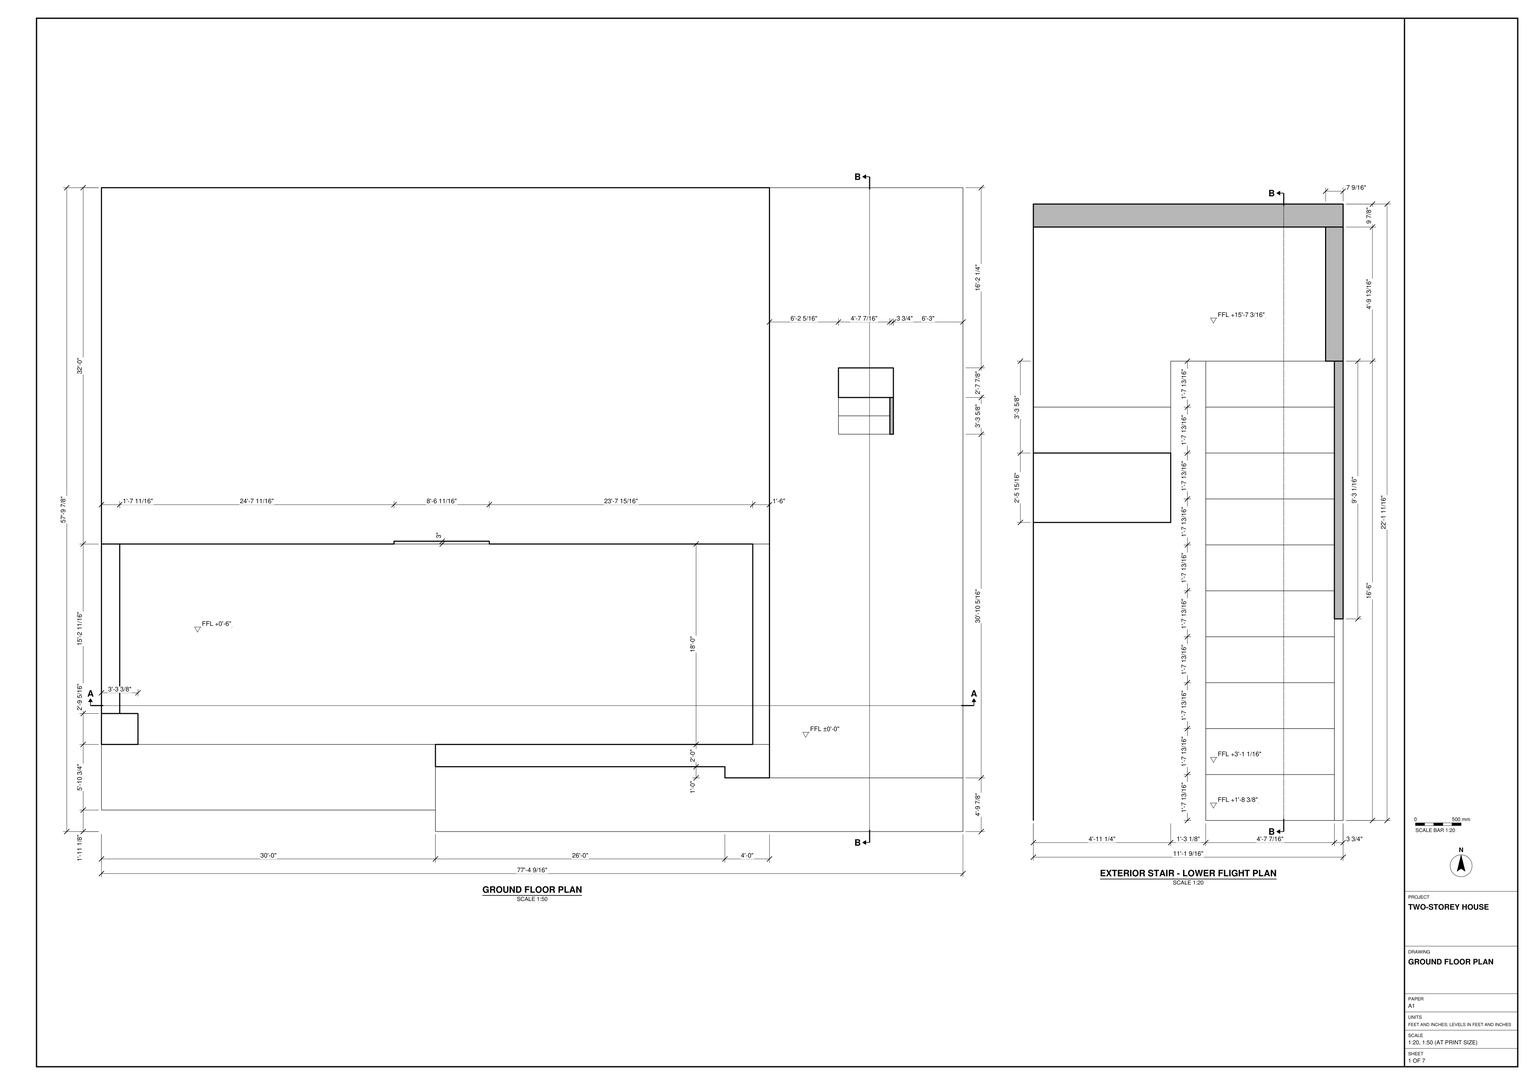
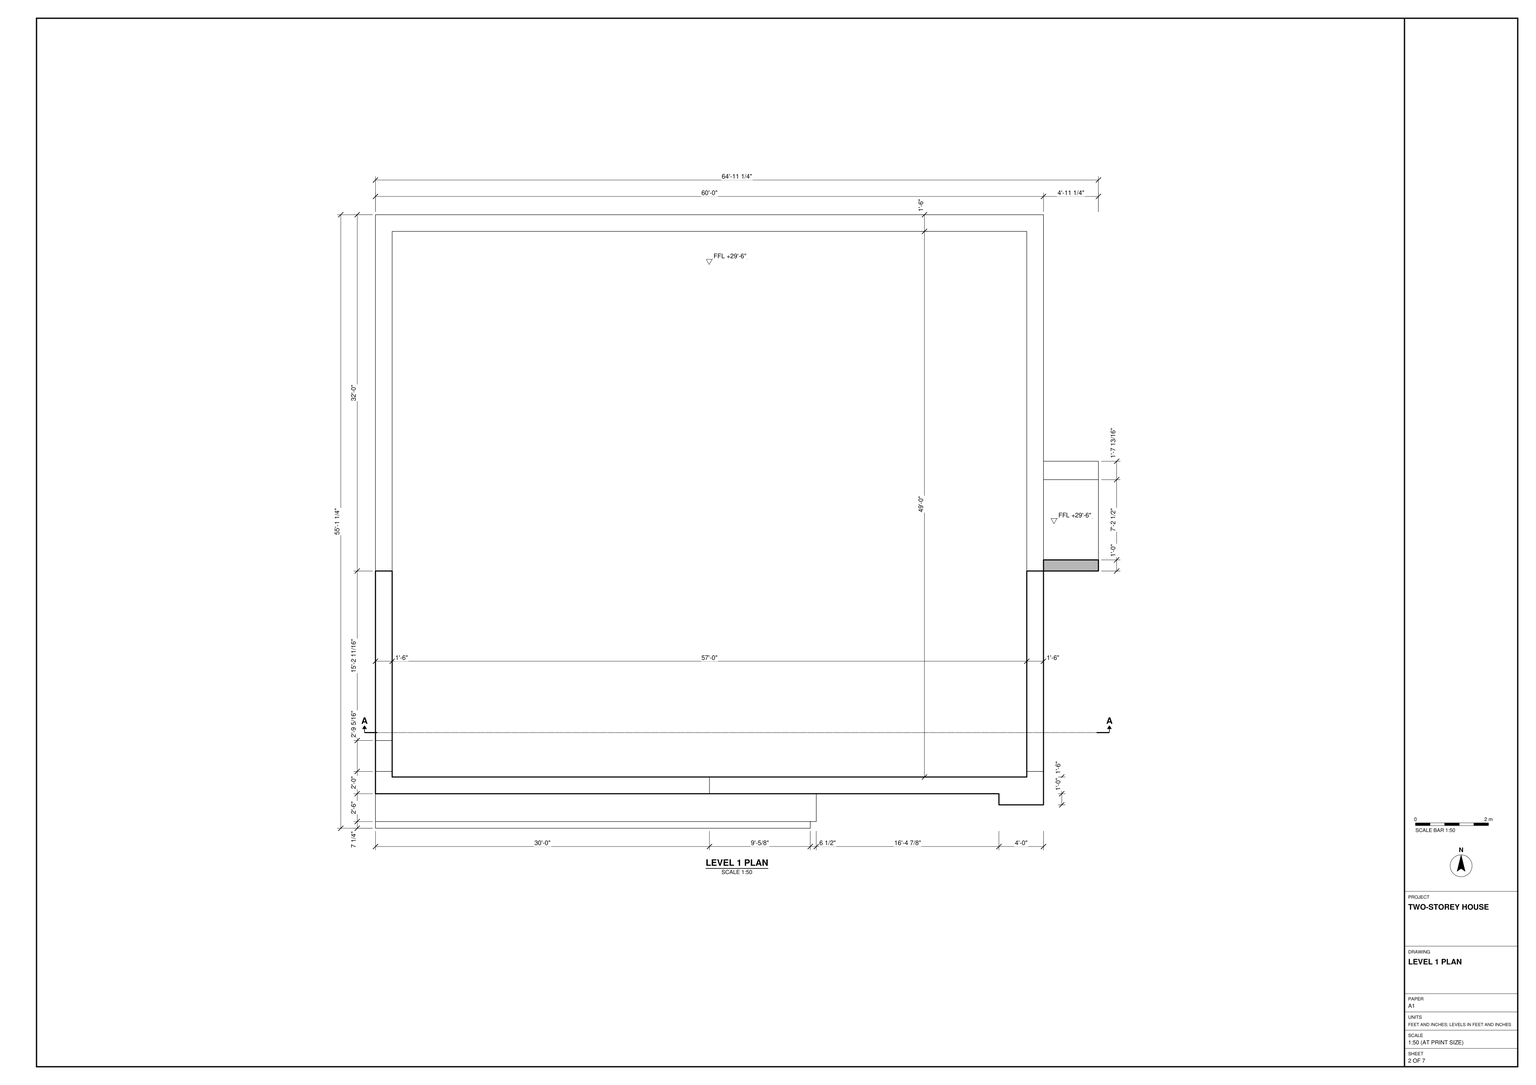
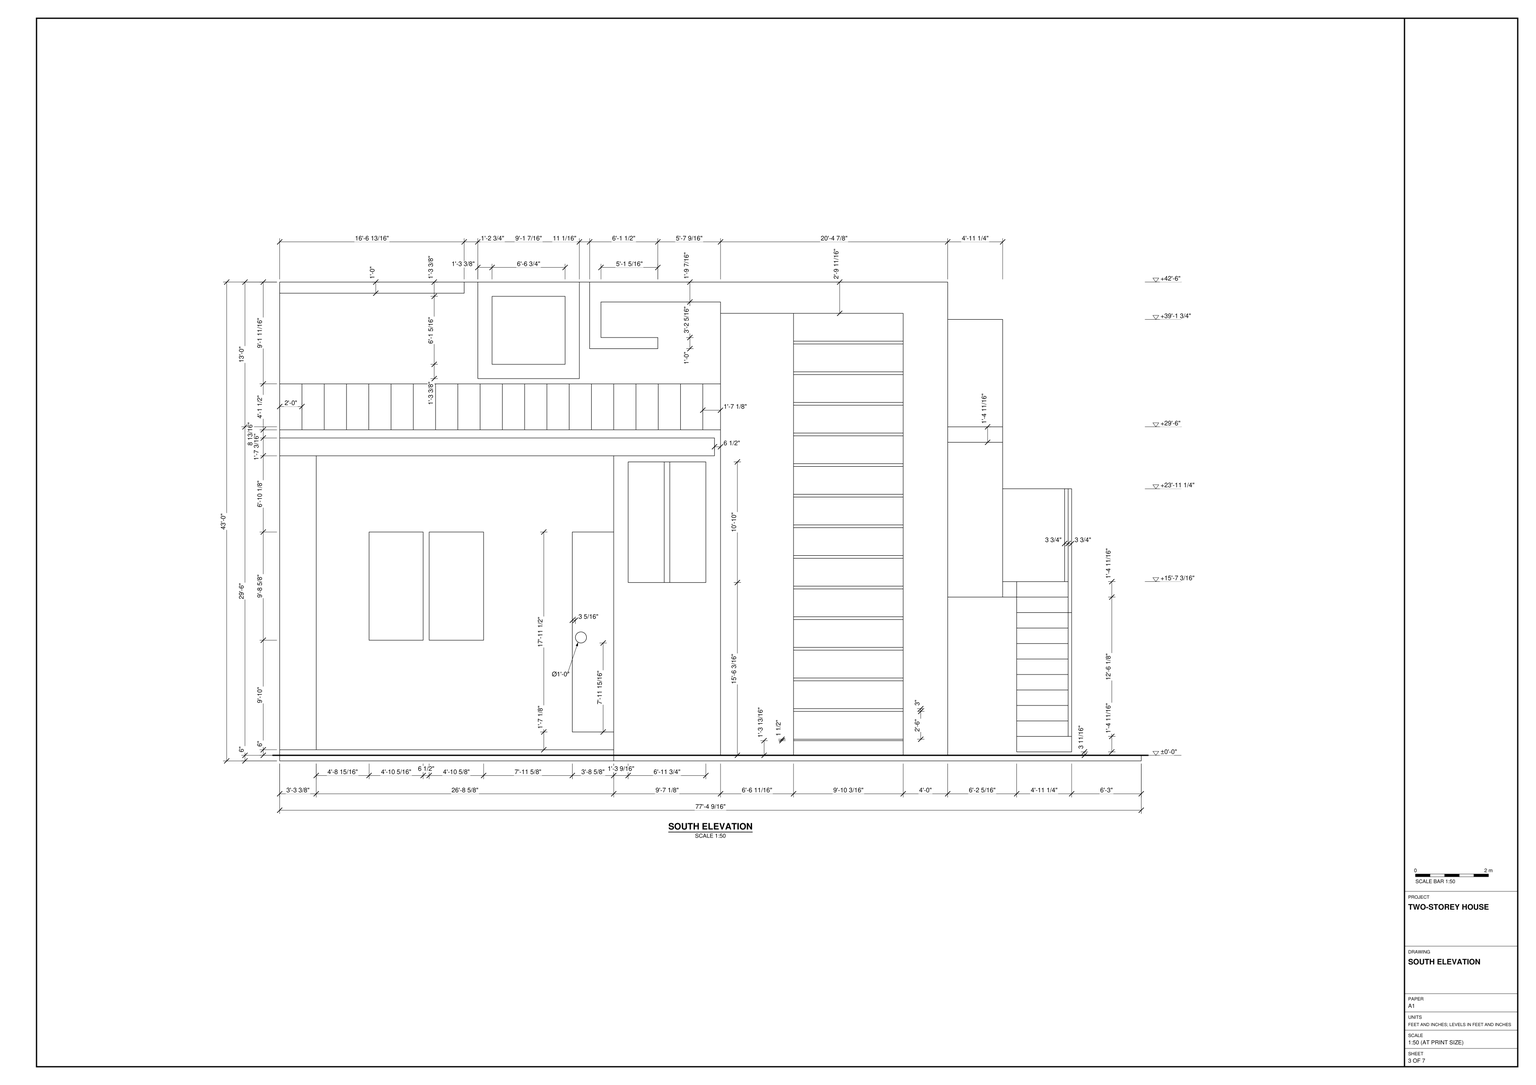
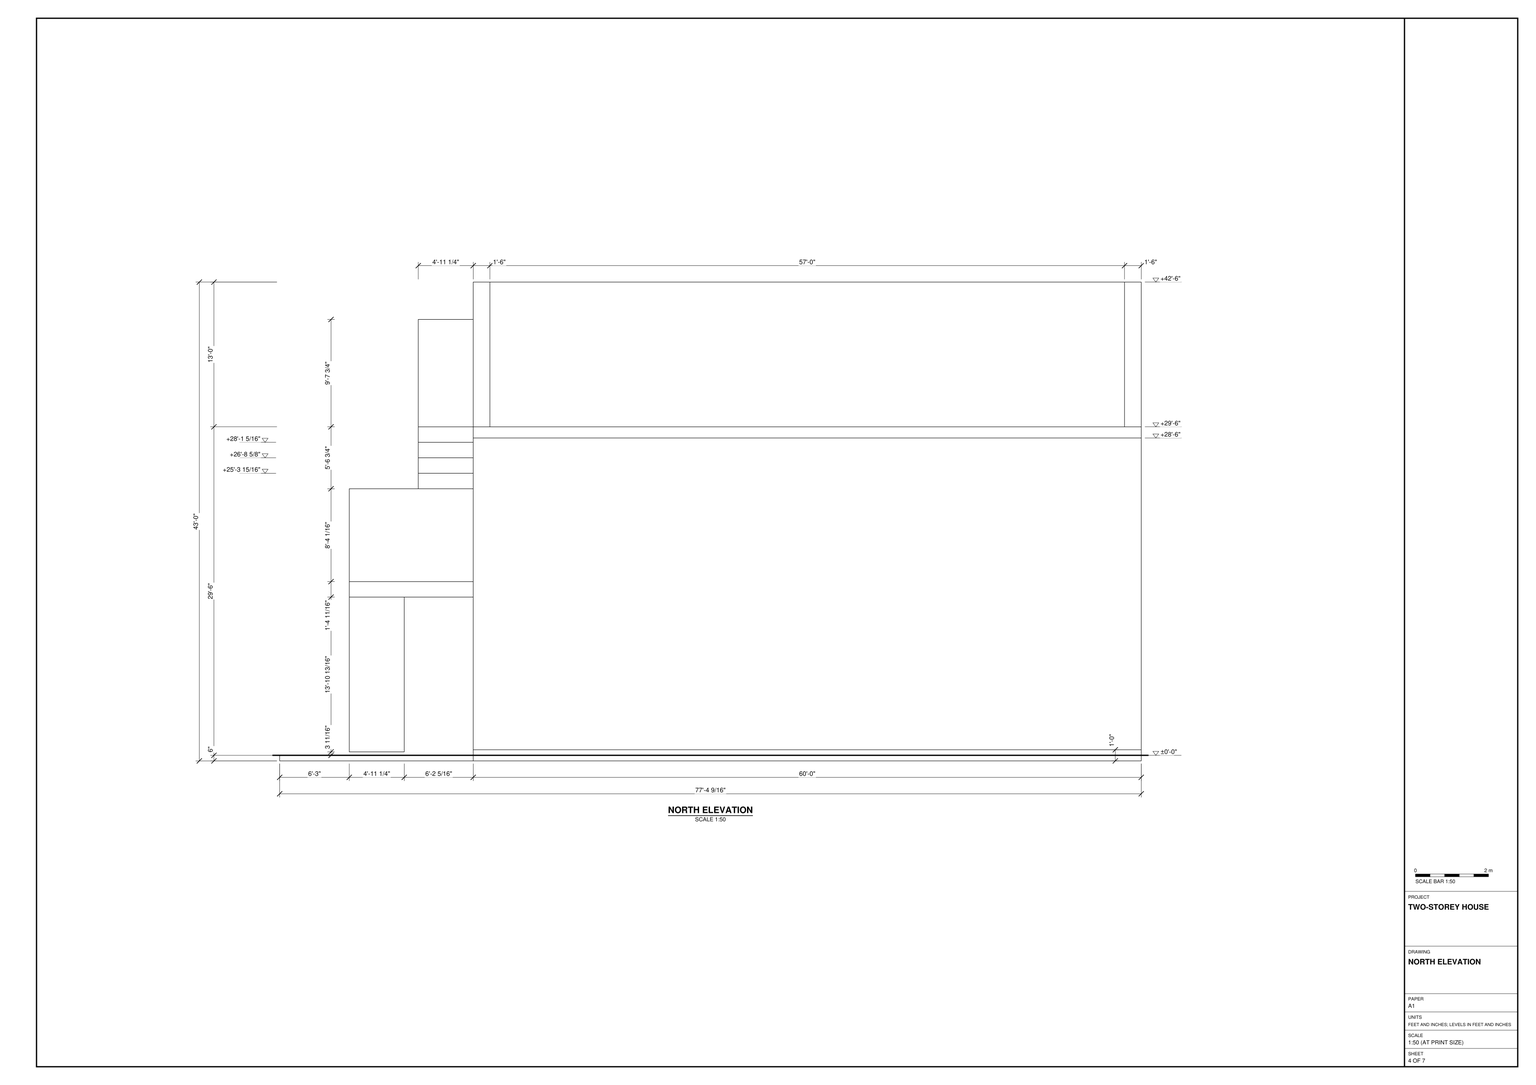
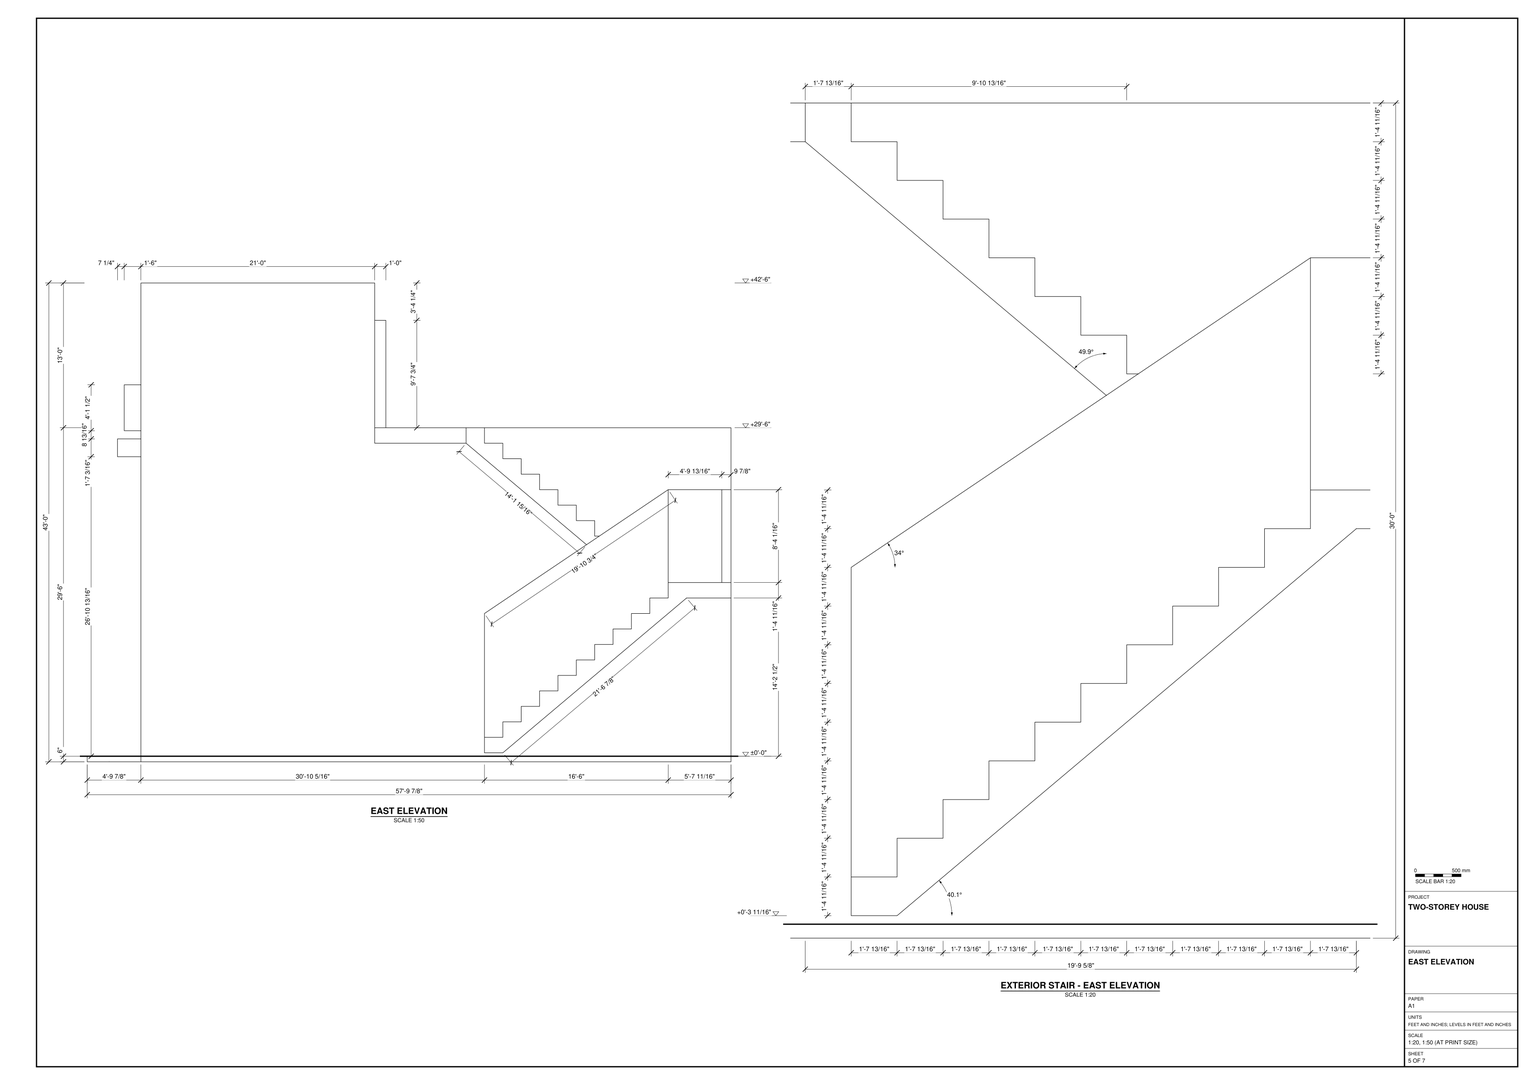
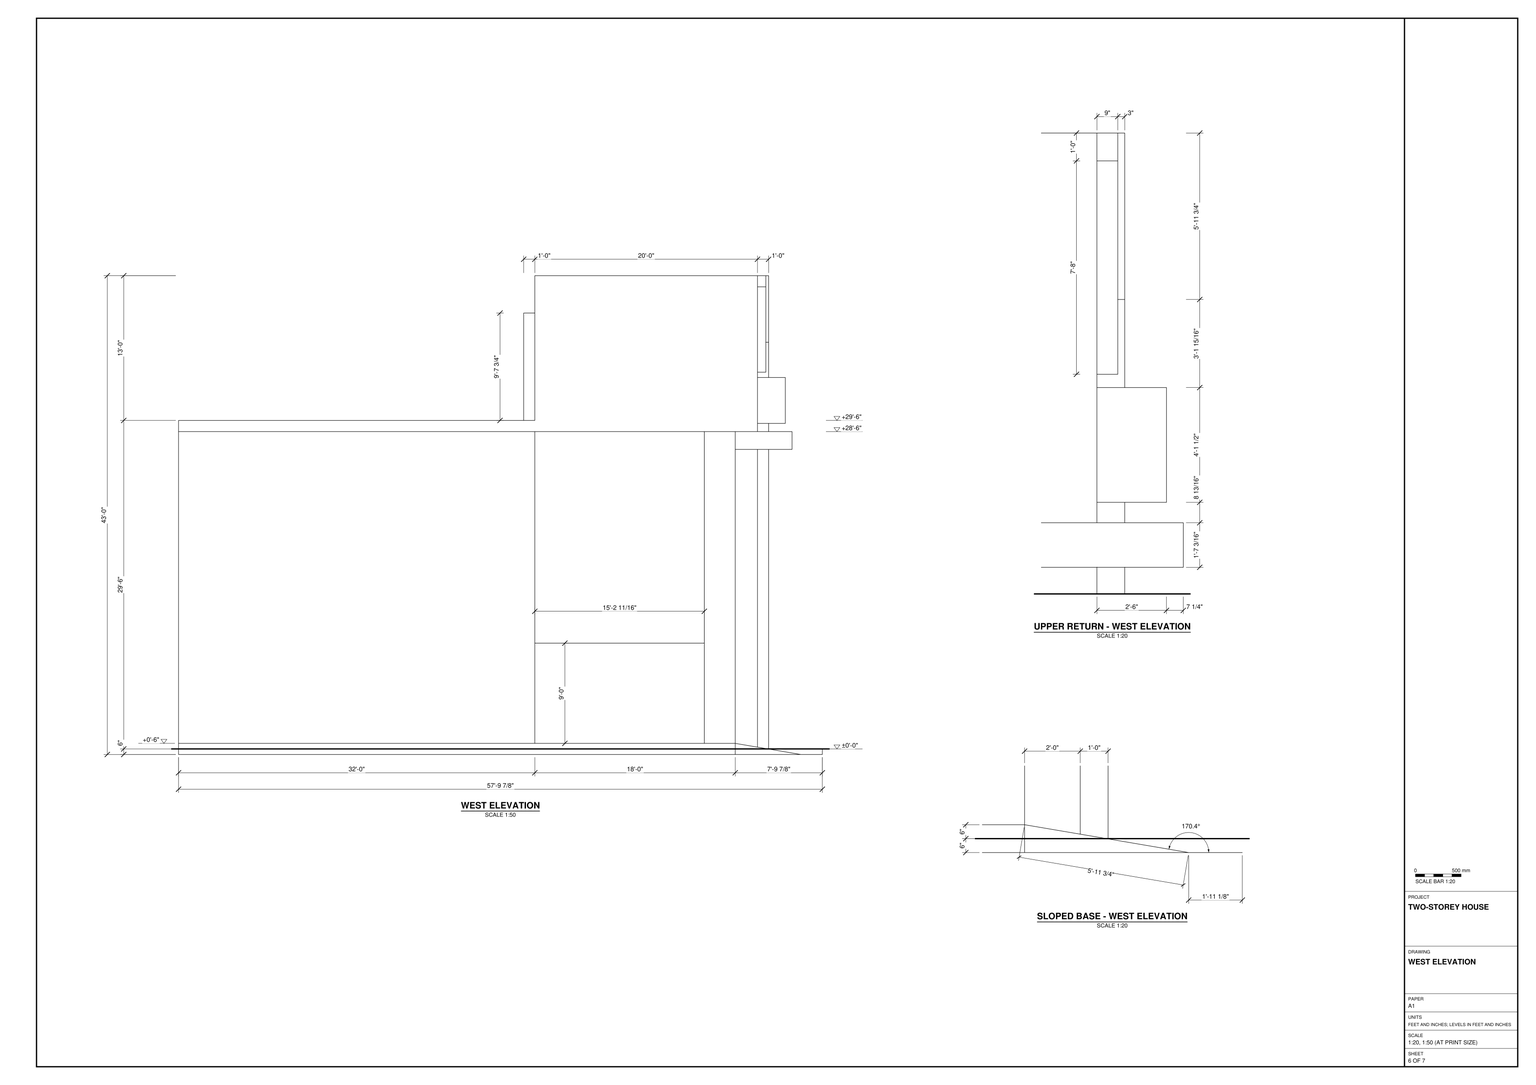
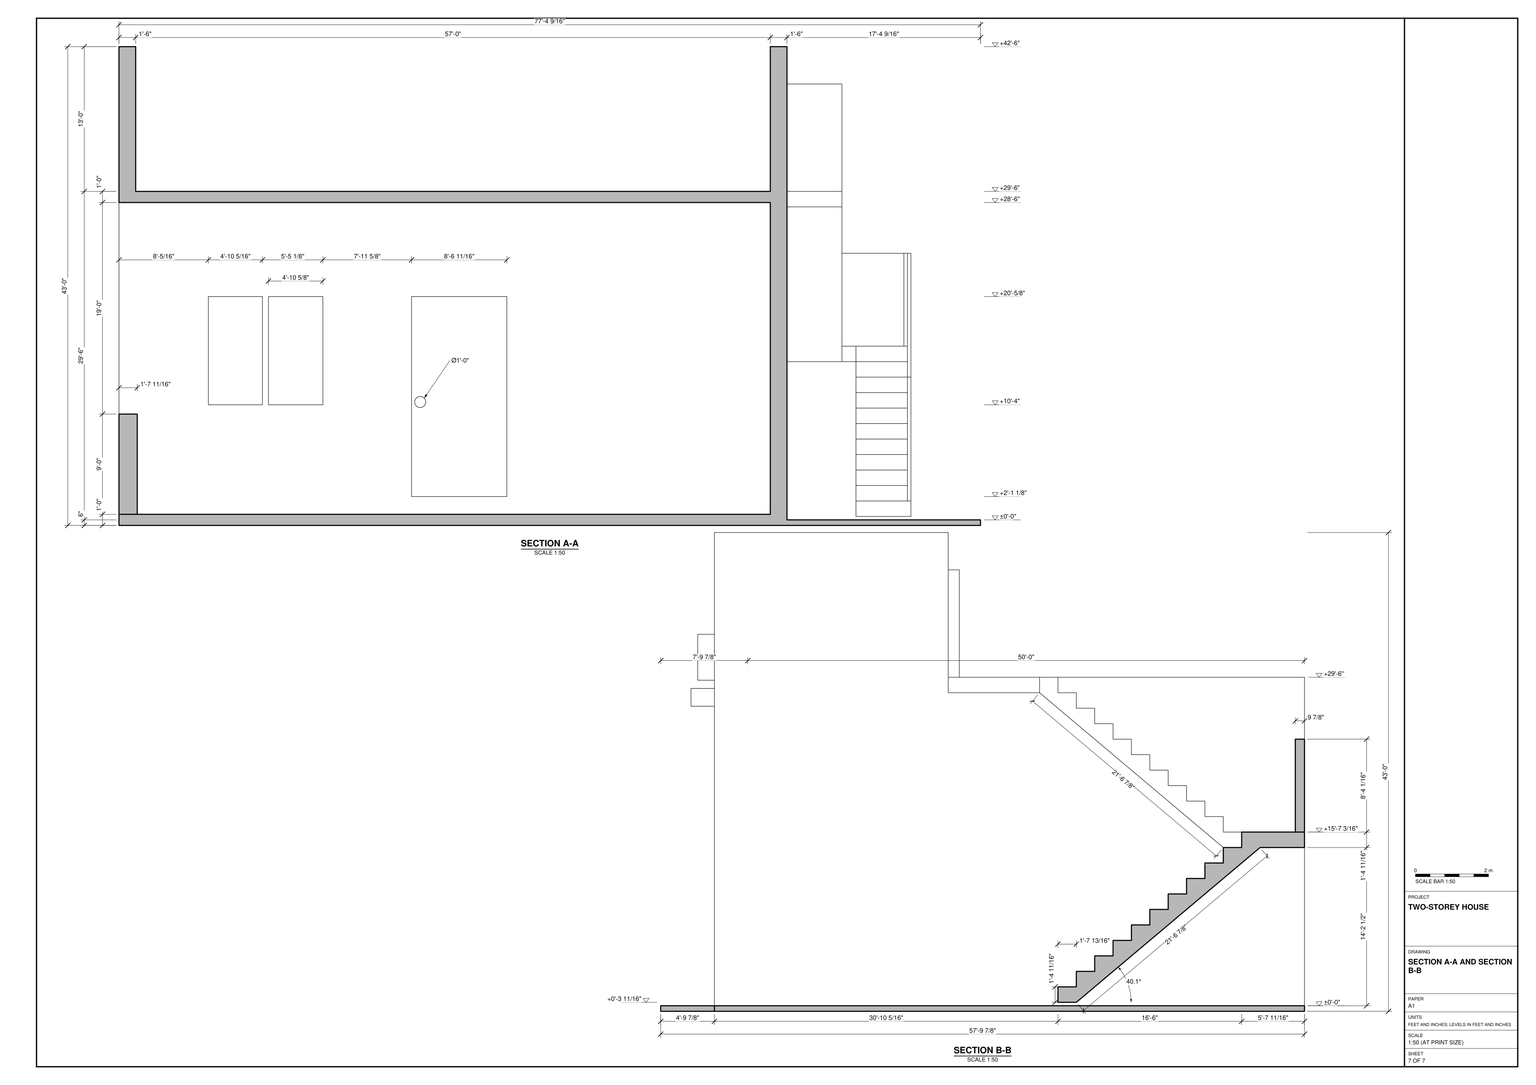
Build the house in SketchUp from task_files/diagram_01.pdf. Work in feet and inches. The overall model, including the base and exterior stair, measures 77'-4 9/16" along X, 57'-9 7/8" along Y and 43'-0" along Z. Set the ground-floor datum at ±0'-0" and the upper floor at +29'-6".

Use the plans to lay out the base, the recessed south frontage and the space beside the house for the stair. Model the walls at their drawn thicknesses and follow the slab edges, offsets and flat roof profile. On the south side, set the entrance wall back behind the outer support and horizontal beam. Place the door and window openings using the elevation, preserving the different sill heights. Model the divided band above the entrance, the square frame and adjoining angular detail near the roofline, and the tall horizontally banded bay toward the stair end of the facade.

Use the stair detail to set out the individual treads, side wall and intermediate landing. Align the return flight with the landing projecting from the upper floor. Keep walls, slabs, stairs and roof in separate groups or components, and group each furniture or joinery piece separately where shown. Use components for repeated parts. Decor and loose items, if shown, may use any suitable library component. Save one SketchUp model as output_files/two_storey_house_with_an_exterior_stair.skp.

# SketchUp Ruby script. Lengths in inches.
U = 1.inch
M = Sketchup.active_model
def pt(a) = Geom::Point3d.new(a.map { |v| v * U })
def face(e, loops, mat)
  f = e.add_face(loops[0].map { |a| pt(a) })
  loops[1..].each { |l| e.add_face(l.map { |a| pt(a) }).erase! }
  f.material = f.back_material = mat if mat
  f
end
# faces: each face lists its corners as indices into pts; further lists are holes
def faces(e, pts, list, mat = nil) = list.each { |f| face(e, (f[0].is_a?(Array) ? f : [f]).map { |l| l.map { |i| pts[i] } }, mat) }
# xy, xz, yz: faces in a plane at the given z, y or x. An outline is a flat list of corners, or four numbers for a rectangle; further outlines are holes
def ring(l) = l.size == 4 ? [[l[0], l[1]], [l[2], l[1]], [l[2], l[3]], [l[0], l[3]]] : l.each_slice(2).to_a
def flat(e, list, mat, &to3) = list.each { |f| face(e, (f[0].is_a?(Array) ? f : [f]).map { |l| ring(l).map { |u, v| to3.(u, v) } }, mat) }
def xy(e, z, list, mat = nil) = flat(e, list, mat) { |x, y| [x, y, z] }
def xz(e, y, list, mat = nil) = flat(e, list, mat) { |x, z| [x, y, z] }
def yz(e, x, list, mat = nil) = flat(e, list, mat) { |y, z| [x, y, z] }
def lines(e, pts, list) = list.each { |a, b| e.add_line(pt(pts[a]), pt(pts[b])) }
# prism: a flat outline (further loops are holes) pulled along v
def prism(e, loops, v, mat = nil)
  f = face(e, loops, mat); d = Geom::Vector3d.new(v.map { |x| x * U })
  f.pushpull(f.normal.samedirection?(d) ? d.length : -d.length)
end
def box(e, o, s, mat = nil) = prism(e, [[o, [o[0] + s[0], o[1], o[2]], [o[0] + s[0], o[1] + s[1], o[2]], [o[0], o[1] + s[1], o[2]]]], [0, 0, s[2]], mat)
def at(x, y, z, deg = 0) = Geom::Transformation.translation(pt([x, y, z])) * Geom::Transformation.rotation(ORIGIN, Z_AXIS, deg.degrees)
def axes(o, x, y, z) = Geom::Transformation.new([*x, 0, *y, 0, *z, 0, *pt(o).to_a, 1])
def part(name) = M.definitions.add(name)
# library, detail: a bought-in or finely detailed component or shape, given as its bounding box
def library(name, o, s) = part(name).tap { |d| box(d.entities, o, s) }
def detail(e, o, s) = box(e.add_group.entities, o, s)
def put(e, d, t, mat = nil) = e.add_instance(d, t).tap { |i| i.material = mat if mat }
def group(e, t, mat = nil) = e.add_group.tap { |g| g.transformation = t; g.material = mat if mat }.entities
root = M.entities
M.materials.add("[0006_Pink]").color = [255, 192, 203]
M.materials.add("[0007_MistyRose]").color = [255, 228, 225]
M.materials.add("[0009_Linen]").color = [250, 240, 230]
M.materials.add("[0018_Brown]").color = [79, 20, 20]
M.materials.add("[0099_LightSteelBlue]").color = [176, 196, 222]
M.materials.add("[0100_SteelBlue]").color = [60, 112, 155]
M.materials.add("[0110_LightSlateGray]").color = [119, 136, 153]
M.materials.add("[0118_Thistle]").color = [216, 191, 216]
M.materials.add("[0119_RosyBrown]").color = [188, 143, 143]
M.materials.add("[0125_Plum]").color = [221, 160, 221]
M.materials.add("[0137_Black]").color = [0, 0, 0]
M.materials.add("[Granite Dark Gray]").color = [69, 68, 68]
M.materials.add("[Grass Dark Green]").color = [106, 157, 55]
M.materials.add("[Stone Coursed Rough]").color = [165, 160, 130]
M.materials.add("[Stone Marble]").color = [143, 138, 136]
M.materials.add("[Translucent Glass Gray]").color = [128, 128, 128]
M.materials["[Translucent Glass Gray]"].alpha = 0.5
xy(root,0,[[360,0,928.5625,57.875],[0,23.125,360,93.875],[672,57.875,672,69.875,360,69.875,360,93.875,0,93.875,0,693.875,928.5625,693.875,928.5625,57.875],[360,57.875,672,69.875]])
xy(root,6,[[720,57.875,928.5625,693.875]])
xy(root,6,[[360,0,928.5625,0,928.5625,57.875,672,57.875,672,69.875,360,69.875]],"[Grass Dark Green]")
xy(root,9.69,[[794.34,428.16,853.56,447.96]])
xy(root,12,[[0,93.875,39.375,127.1875],[0,127.1875,19.6875,309.875]])
xy(root,12,[[39.375,93.875,702,93.875,702,309.875,19.6875,309.875,19.6875,127.1875,39.375,127.1875]],"[Stone Marble]")
xy(root,26.37,[[849.78,428.16,853.56,447.96]])
xy(root,26.37,[[794.34,428.16,849.78,447.96]],"[Granite Dark Gray]")
xy(root,31.15,[[315.37,309.875,418.06,312.875]])
xy(root,43.05,[[849.78,447.96,853.56,467.76]])
xy(root,43.05,[[794.34,447.96,849.78,467.76]],"[Granite Dark Gray]")
xy(root,59.73,[[849.78,467.76,853.56,487.56]])
xy(root,59.73,[[794.34,467.76,849.78,487.56]],"[Granite Dark Gray]")
xy(root,76.42,[[849.78,487.56,853.56,507.36]])
xy(root,76.42,[[794.34,487.56,849.78,507.36]],"[Granite Dark Gray]")
xy(root,93.1,[[849.78,507.36,853.56,527.16]])
xy(root,93.1,[[794.34,507.36,849.78,527.16]],"[Granite Dark Gray]")
xy(root,109.78,[[849.78,527.16,853.56,546.96]])
xy(root,109.78,[[794.34,527.16,849.78,546.96]],"[Granite Dark Gray]")
xy(root,120,[[0,127.1875,19.6875,309.875]])
xy(root,126.46,[[849.78,546.96,853.56,566.76]])
xy(root,126.46,[[794.34,546.96,849.78,566.76]],"[Granite Dark Gray]")
xy(root,130.02,[[96.32,309.875,154.63,311.875],[161.1,309.875,219.76,311.875]],"[0137_Black]")
xy(root,143.14,[[849.78,566.76,853.56,586.56]])
xy(root,143.14,[[794.34,566.76,849.78,586.56]],"[Granite Dark Gray]")
xy(root,159.82,[[849.78,586.56,853.56,606.36]])
xy(root,159.82,[[794.34,586.56,849.78,606.36]],"[Granite Dark Gray]")
xy(root,176.5,[[720,606.36,720,693.875,794.34,693.875,794.34,626.16,779.22,626.16,779.22,606.36],[849.78,606.36,853.56,626.16],[794.34,645.96,853.56,693.875]])
xy(root,176.5,[[794.34,606.36,849.78,626.16]],"[Granite Dark Gray]")
xy(root,192.21,[[375.57,69.875,414.44,71.875],[420.44,69.875,459.32,71.875]])
xy(root,193.1875,[[846,626.16,853.56,683.98],[720,683.97,720,693.875,853.56,693.875,853.56,683.98,846,683.98]])
xy(root,193.1875,[[720,606.36,779.22,606.36,779.22,626.16,846,626.16,846,683.98,720,683.97]],"[Granite Dark Gray]")
xy(root,209.87,[[720,586.56,779.22,606.36]],"[Granite Dark Gray]")
xy(root,226.55,[[720,566.76,779.22,586.56]],"[Granite Dark Gray]")
xy(root,243.23,[[720,546.96,779.22,566.76]],"[Granite Dark Gray]")
xy(root,246.65,[[315.37,309.875,418.06,312.875]])
xy(root,246.65,[[96.32,309.875,154.63,311.875],[161.1,309.875,219.76,311.875]],"[0137_Black]")
xy(root,259.91,[[720,527.16,779.22,546.96]],"[Granite Dark Gray]")
xy(root,276.59,[[720,507.36,779.22,527.16]],"[Granite Dark Gray]")
xy(root,293.27,[[846,626.16,853.56,683.98],[720,683.97,846,683.98,853.56,683.98,853.56,693.875,720,693.875]],"[0009_Linen]")
xy(root,293.27,[[720,487.56,779.22,507.36]],"[Granite Dark Gray]")
xy(root,309.96,[[720,467.76,779.22,487.56]],"[Granite Dark Gray]")
xy(root,322.21,[[375.57,69.875,414.44,71.875],[420.44,69.875,459.32,71.875]])
xy(root,326.64,[[720,447.96,779.22,467.76]],"[Granite Dark Gray]")
xy(root,328.8,[[0,32.625,0,93.875,360,93.875,360,69.875,468.625,69.875,468.625,32.625]],"[0125_Plum]")
xy(root,343.32,[[720,309.875,779.22,408.36]])
xy(root,343.32,[[720,428.16,779.22,447.96]],"[Granite Dark Gray]")
xy(root,348,[[0,69.875,360,93.875],[39.375,93.875,39.375,127.1875,0,127.1875,0,309.875,702,309.875,702,93.875]])
xy(root,348,[[0,32.625,468.625,69.875]],"[0125_Plum]")
xy(root,356.81,[[0,39.875,475.125,69.875]],"[0099_LightSteelBlue]")
xy(root,360,[[18,87.875,702,675.875],[0,309.875,18,309.875,18,675.875,702,675.875,702,309.875,720,309.875,720,693.875,0,693.875],[720,309.875,779.22,321.875]])
xy(root,360,[[720,321.875,779.22,408.36]],"[0009_Linen]")
xy(root,360,[[720,408.36,779.22,428.16]],"[Granite Dark Gray]")
xy(root,406.29,[[0,39.875,475.125,69.875]],"[0099_LightSteelBlue]")
xy(root,412,[[213.55,60.875,322.98,69.875]],"[0100_SteelBlue]")
xy(root,427.35,[[228.9,60.875,307.63,69.875]],"[0100_SteelBlue]")
xy(root,444.25,[[334.0625,57.875,407.57,69.875]],"[0006_Pink]")
xy(root,456.25,[[346.25,57.875,407.57,69.875]],"[0006_Pink]")
xy(root,475.75,[[720,309.875,779.22,321.875]],"[0009_Linen]")
xy(root,482.3125,[[475.125,57.875,672,69.875]],"[0006_Pink]")
xy(root,494.5625,[[346.1875,57.875,346.25,69.875]])
xy(root,494.5625,[[346.25,57.875,475.125,69.875]],"[0006_Pink]")
xy(root,500.65,[[228.9,60.875,307.63,69.875]])
xy(root,504,[[0,60.875,198.8125,69.875]],"[0110_LightSlateGray]")
xy(root,516,[[0,60.875,198.8125,69.875]])
xy(root,516,[[334.0625,57.875,720,57.875,720,309.875,702,309.875,702,87.875,18,87.875,18,309.875,0,309.875,0,69.875,334.0625,69.875]],"[0006_Pink]")
xy(root,516,[[213.55,60.875,322.98,69.875]],"[0100_SteelBlue]")
xz(root,0,[[360,0,928.5625,6]],"[Grass Dark Green]")
xz(root,32.625,[[0,328.8,468.625,348]],"[0125_Plum]")
xz(root,39.875,[[0,356.81,24,406.29],[24,356.81,48,406.29],[48,356.81,72,406.29],[72,356.81,96,406.29],[96,356.81,120,406.29],
  [120,356.81,144,406.29],[144,356.81,168,406.29],[168,356.81,192,406.29],[192,356.81,216,406.29],[216,356.81,240,406.29],
  [240,356.81,264,406.29],[264,356.81,288,406.29],[288,356.81,312,406.29],[312,356.81,336,406.29],[336,356.81,360,406.29],
  [360,356.81,384,406.29],[384,356.81,408,406.29],[408,356.81,432,406.29],[432,356.81,456,406.29],[456,356.81,475.125,406.29]],"[0099_LightSteelBlue]")
xz(root,57.875,[[672,0,720,6],[720,0,928.5625,6]])
xz(root,57.875,[[672,6,720,6,720,516,334.0625,516,334.0625,444.25,407.57,444.25,407.57,456.25,346.25,456.25,346.25,494.5625,475.125,494.5625,475.125,482.3125,672,482.3125]],"[0006_Pink]")
xz(root,60.875,[[[213.55,412,322.98,516],[228.9,427.35,307.63,500.65]]],"[0100_SteelBlue]")
xz(root,60.875,[[0,504,198.8125,516]],"[0110_LightSlateGray]")
xz(root,69.875,[[360,0,475.125,6],[475.125,0,553.8125,6],[553.8125,0,672,6],[553.8125,21.8125,672,23.3125],[553.8125,53.3125,672,56.3125],
  [553.8125,86.3125,672,89.3125],[553.8125,119.3125,672,122.3125],[553.8125,152.3125,672,155.3125],[553.8125,185.3125,672,188.3125],[414.44,192.21,420.44,322.21],
  [553.8125,218.3125,672,221.3125],[553.8125,251.3125,672,254.3125],[553.8125,284.3125,672,287.3125],[553.8125,317.3125,672,320.3125],[553.8125,350.3125,672,353.3125],
  [0,356.81,475.125,406.29],[553.8125,383.3125,672,386.3125],[[213.55,412,322.98,516],[228.9,427.35,307.63,500.65]],[553.8125,416.3125,672,419.3125],[228.9,427.35,307.63,500.65],
  [553.8125,449.3125,672,452.3125],[0,504,198.8125,516]])
xz(root,69.875,[[553.8125,6,672,21.8125],[553.8125,23.3125,672,53.3125],[553.8125,56.3125,672,86.3125],[553.8125,89.3125,672,119.3125],[553.8125,122.3125,672,152.3125],
  [553.8125,155.3125,672,185.3125],[553.8125,188.3125,672,218.3125],[553.8125,221.3125,672,251.3125],[553.8125,254.3125,672,284.3125],[553.8125,287.3125,672,317.3125],
  [553.8125,320.3125,672,350.3125],[553.8125,353.3125,672,383.3125],[553.8125,386.3125,672,416.3125],[553.8125,419.3125,672,449.3125],[553.8125,452.3125,672,482.3125]],"[0119_RosyBrown]")
xz(root,69.875,[[[360,6,475.125,6,475.125,356.81,0,356.81,0,348,468.625,348,468.625,328.8,360,328.8],[375.57,192.21,459.32,322.21]],[475.125,6,553.8125,482.3125],[0,406.29,475.125,406.29,475.125,494.5625,346.25,494.5625,346.25,456.25,407.57,456.25,407.57,444.25,334.0625,444.25,334.0625,516,322.98,516,322.98,412,213.55,412,213.55,516,198.8125,516,198.8125,504,0,504]],"[0125_Plum]")
xz(root,71.875,[[375.57,192.21,414.44,322.21],[420.44,192.21,459.32,322.21]],"[Translucent Glass Gray]")
xz(root,87.875,[[18,360,702,516]])
xz(root,93.875,[[0,0,360,12],[360,12,360,328.8,39.375,328.8,39.375,348,702,348,702,12],[0,328.8,39.375,348]])
xz(root,93.875,[[0,12,39.375,328.8]],"[Stone Coursed Rough]")
xz(root,127.1875,[[0,12,19.6875,120],[19.6875,12,19.6875,120,0,120,0,348,39.375,348,39.375,12]])
xz(root,309.875,[[0,12,19.6875,120],[324.59,127.05,326.15,127.23,327.61,127.8125,328.86,128.74,329.84,129.97,330.46,131.41,330.6875,132.96,330.51,134.52,329.93,135.97,329,137.23,327.77,138.2,326.33,138.82,324.78,139.05,323.22,138.87,321.77,138.29,320.51,137.36,319.54,136.13,318.92,134.7,318.6875,133.15,318.87,131.59,319.45,130.13,320.38,128.875,321.61,127.9,323.05,127.28],[0,360,18,516],[702,360,720,516]])
xz(root,309.875,[[720,343.32,779.22,360],[720,360,779.22,475.75]],"[0009_Linen]")
xz(root,309.875,[[[19.6875,12,702,12,702,348,0,348,0,120,19.6875,120],[315.37,31.15,418.06,246.65],[161.1,130.02,219.76,246.65],[96.32,130.02,154.63,246.65]]],"[Stone Coursed Rough]")
xz(root,311.875,[[96.32,130.02,154.63,246.65],[161.1,130.02,219.76,246.65]],"[Translucent Glass Gray]")
xz(root,312.875,[[[315.37,31.15,418.06,246.65],[324.59,127.05,323.05,127.28,321.61,127.9,320.38,128.875,319.45,130.13,318.87,131.59,318.6875,133.15,318.92,134.7,319.54,136.13,320.51,137.36,321.77,138.29,323.22,138.87,324.78,139.05,326.33,138.82,327.77,138.2,329,137.23,329.93,135.97,330.51,134.52,330.6875,132.96,330.46,131.41,329.84,129.97,328.86,128.74,327.61,127.8125,326.15,127.23]]],"[0018_Brown]")
xz(root,321.875,[[720,360,779.22,475.75]],"[0009_Linen]")
xz(root,408.36,[[720,343.32,779.22,360]])
xz(root,428.16,[[849.78,26.37,853.56,159.82]])
xz(root,428.16,[[794.34,9.69,853.56,26.37],[720,343.32,779.22,360]],"[Granite Dark Gray]")
xz(root,447.96,[[849.78,26.37,853.56,43.05]])
xz(root,447.96,[[794.34,26.37,849.78,43.05],[720,326.64,779.22,343.32]],"[Granite Dark Gray]")
xz(root,467.76,[[849.78,43.05,853.56,59.73]])
xz(root,467.76,[[794.34,43.05,849.78,59.73],[720,309.96,779.22,326.64]],"[Granite Dark Gray]")
xz(root,487.56,[[849.78,59.73,853.56,76.42]])
xz(root,487.56,[[794.34,59.73,849.78,76.42],[720,293.27,779.22,309.96]],"[Granite Dark Gray]")
xz(root,507.36,[[849.78,76.42,853.56,93.1]])
xz(root,507.36,[[794.34,76.42,849.78,93.1],[720,276.59,779.22,293.27]],"[Granite Dark Gray]")
xz(root,527.16,[[849.78,93.1,853.56,109.78]])
xz(root,527.16,[[794.34,93.1,849.78,109.78],[720,259.91,779.22,276.59]],"[Granite Dark Gray]")
xz(root,546.96,[[849.78,109.78,853.56,126.46]])
xz(root,546.96,[[794.34,109.78,849.78,126.46],[720,243.23,779.22,259.91]],"[Granite Dark Gray]")
xz(root,566.76,[[849.78,126.46,853.56,143.14]])
xz(root,566.76,[[794.34,126.46,849.78,143.14],[720,226.55,779.22,243.23]],"[Granite Dark Gray]")
xz(root,586.56,[[849.78,143.14,853.56,159.82]])
xz(root,586.56,[[794.34,143.14,849.78,159.82],[720,209.87,779.22,226.55]],"[Granite Dark Gray]")
xz(root,606.36,[[849.78,159.82,853.56,176.5]])
xz(root,606.36,[[794.34,159.82,849.78,176.5],[720,193.1875,779.22,209.87]],"[Granite Dark Gray]")
xz(root,626.16,[[849.78,176.5,853.56,193.1875],[849.78,193.1875,853.56,293.27]])
xz(root,626.16,[[779.22,176.5,794.34,193.1875],[846,193.1875,849.78,293.27]],"[0009_Linen]")
xz(root,626.16,[[794.34,176.5,849.78,193.1875]],"[Granite Dark Gray]")
xz(root,683.98,[[846,193.1875,853.56,293.27]])
xz(root,693.875,[[0,0,720,12],[720,0,928.5625,6],[0,12,720,348],[720,176.5,853.56,193.1875],[0,348,720,360]])
xz(root,693.875,[[720,193.1875,853.56,293.27]],"[0009_Linen]")
yz(root,0,[[23.125,0,93.875,12,93.875,0],[93.875,0,693.875,12],[309.875,12,693.875,348],[69.875,348,69.875,516,309.875,516,309.875,360,693.875,360,693.875,348],[60.875,504,69.875,516]])
yz(root,0,[[39.875,356.81,69.875,406.29]],"[0099_LightSteelBlue]")
yz(root,0,[[32.625,328.8,93.875,348]],"[0125_Plum]")
yz(root,0,[[93.875,12,127.1875,348],[127.1875,12,309.875,120]],"[Stone Coursed Rough]")
yz(root,18,[[87.875,360,111.875,516],[111.875,360,309.875,516]])
yz(root,19.6875,[[127.1875,12,309.875,120]],"[Stone Coursed Rough]")
yz(root,39.375,[[93.875,12,127.1875,348]],"[Stone Coursed Rough]")
yz(root,96.32,[[309.875,130.02,311.875,246.65]],"[0137_Black]")
yz(root,154.63,[[309.875,130.02,311.875,246.65]],"[0137_Black]")
yz(root,161.1,[[309.875,130.02,311.875,246.65]],"[0137_Black]")
yz(root,198.8125,[[60.875,504,69.875,516]],"[0110_LightSlateGray]")
yz(root,213.55,[[60.875,412,69.875,516]],"[0100_SteelBlue]")
yz(root,219.76,[[309.875,130.02,311.875,246.65]],"[0137_Black]")
yz(root,228.9,[[60.875,427.35,69.875,500.65]],"[0100_SteelBlue]")
yz(root,307.63,[[60.875,427.35,69.875,500.65]],"[0100_SteelBlue]")
yz(root,315.37,[[309.875,31.15,312.875,246.65]])
yz(root,322.98,[[60.875,412,69.875,516]],"[0100_SteelBlue]")
yz(root,334.0625,[[57.875,444.25,69.875,516]],"[0006_Pink]")
yz(root,346.25,[[57.875,456.25,69.875,494.5625]],"[0006_Pink]")
yz(root,360,[[0,0,0,6,58.5,6,23.125,0],[23.125,0,58.5,6,69.875,6,69.875,0],[69.875,0,93.875,0,93.875,12,69.875,7.93],[58.5,6,69.875,6,69.875,7.93]])
yz(root,360,[[69.875,7.93,69.875,328.8,93.875,328.8,93.875,12]],"[0118_Thistle]")
yz(root,375.57,[[69.875,192.21,71.875,322.21]])
yz(root,407.57,[[57.875,444.25,69.875,456.25]],"[0006_Pink]")
yz(root,414.44,[[69.875,192.21,71.875,322.21]])
yz(root,418.06,[[309.875,31.15,312.875,246.65]])
yz(root,420.44,[[69.875,192.21,71.875,322.21]])
yz(root,459.32,[[69.875,192.21,71.875,322.21]])
yz(root,468.625,[[32.625,328.8,69.875,348]],"[0125_Plum]")
yz(root,475.125,[[57.875,482.3125,69.875,494.5625]],"[0006_Pink]")
yz(root,475.125,[[39.875,356.81,69.875,406.29]],"[0099_LightSteelBlue]")
yz(root,672,[[57.875,0,69.875,6]])
yz(root,672,[[57.875,6,69.875,482.3125]],"[0006_Pink]")
yz(root,702,[[93.875,12,309.875,348],[87.875,360,93.875,516],[93.875,360,111.875,516],[111.875,360,309.875,516]])
yz(root,720,[[606.36,176.5,408.36,343.32,408.36,360,428.16,360,428.16,343.32,447.96,343.32,447.96,326.64,467.76,326.64,467.76,309.96,487.56,309.96,487.56,293.27,507.36,293.27,507.36,276.59,527.16,276.59,527.16,259.91,546.96,259.91,546.96,243.23,566.76,243.23,566.76,226.55,586.56,226.55,586.56,209.87,606.36,209.87,606.36,193.1875,693.875,193.1875,693.875,176.5],[683.97,193.1875,693.875,293.27],[309.875,343.32,408.36,360],[309.875,360,321.875,475.75]])
yz(root,720,[[57.875,6,693.875,6,693.875,176.5,606.36,176.5,408.36,343.32,309.875,343.32,309.875,516,57.875,516]],"[0007_MistyRose]")
yz(root,720,[[606.36,193.1875,683.97,193.1875,683.97,293.27,693.875,293.27,693.875,360,428.16,360,428.16,343.32,447.96,343.32,447.96,326.64,467.76,326.64,467.76,309.96,487.56,309.96,487.56,293.27,507.36,293.27,507.36,276.59,527.16,276.59,527.16,259.91,546.96,259.91,546.96,243.23,566.76,243.23,566.76,226.55,586.56,226.55,586.56,209.87,606.36,209.87]],"[0009_Linen]")
yz(root,779.22,[[309.875,343.32,408.36,360],[309.875,360,321.875,475.75]],"[0009_Linen]")
yz(root,779.22,[[606.36,176.5,626.16,176.5,626.16,193.1875,606.36,193.1875,606.36,209.87,586.56,209.87,586.56,226.55,566.76,226.55,566.76,243.23,546.96,243.23,546.96,259.91,527.16,259.91,527.16,276.59,507.36,276.59,507.36,293.27,487.56,293.27,487.56,309.96,467.76,309.96,467.76,326.64,447.96,326.64,447.96,343.32,428.16,343.32,428.16,360,408.36,360,408.36,343.32]],"[Granite Dark Gray]")
yz(root,794.34,[[428.16,9.69,428.16,26.37,447.96,26.37,447.96,43.05,467.76,43.05,467.76,59.73,487.56,59.73,487.56,76.42,507.36,76.42,507.36,93.1,527.16,93.1,527.16,109.78,546.96,109.78,546.96,126.46,566.76,126.46,566.76,143.14,586.56,143.14,586.56,159.82,606.36,159.82,606.36,176.5,645.96,176.5,447.96,9.69]])
yz(root,846,[[626.16,193.1875,683.98,293.27]],"[0009_Linen]")
yz(root,849.78,[[428.16,26.37,428.16,159.82,626.16,293.27,626.16,176.5,606.36,176.5,606.36,159.82,586.56,159.82,586.56,143.14,566.76,143.14,566.76,126.46,546.96,126.46,546.96,109.78,527.16,109.78,527.16,93.1,507.36,93.1,507.36,76.42,487.56,76.42,487.56,59.73,467.76,59.73,467.76,43.05,447.96,43.05,447.96,26.37]],"[0009_Linen]")
yz(root,853.56,[[428.16,9.69,447.96,9.69,645.96,176.5,693.875,176.5,693.875,193.1875,626.16,193.1875,626.16,176.5,606.36,176.5,606.36,159.82,586.56,159.82,586.56,143.14,566.76,143.14,566.76,126.46,546.96,126.46,546.96,109.78,527.16,109.78,527.16,93.1,507.36,93.1,507.36,76.42,487.56,76.42,487.56,59.73,467.76,59.73,467.76,43.05,447.96,43.05,447.96,26.37,428.16,26.37],[428.16,26.37,447.96,26.37,447.96,43.05,467.76,43.05,467.76,59.73,487.56,59.73,487.56,76.42,507.36,76.42,507.36,93.1,527.16,93.1,527.16,109.78,546.96,109.78,546.96,126.46,566.76,126.46,566.76,143.14,586.56,143.14,586.56,159.82,606.36,159.82,606.36,176.5,626.16,176.5,626.16,293.27,428.16,159.82],[626.16,193.1875,683.98,293.27],[683.98,193.1875,693.875,293.27]],"[0009_Linen]")
yz(root,928.5625,[[0,0,57.875,6],[57.875,0,693.875,6]])
p = [[0,93.875,12],[0,23.125,0],[360,23.125,0],[360,58.5,6],[360,69.875,7.93],[360,93.875,12],
  [39.375,93.875,12],[794.34,447.96,9.69],[794.34,645.96,176.5],[853.56,645.96,176.5],[853.56,447.96,9.69],[324.59,309.875,127.05],
  [323.05,309.875,127.28],[323.05,312.875,127.28],[324.59,312.875,127.05],[326.15,309.875,127.23],[326.15,312.875,127.23],[327.61,309.875,127.8125],
  [327.61,312.875,127.8125],[321.61,309.875,127.9],[321.61,312.875,127.9],[328.86,309.875,128.74],[328.86,312.875,128.74],[320.38,309.875,128.875],
  [320.38,312.875,128.875],[329.84,309.875,129.97],[329.84,312.875,129.97],[319.45,309.875,130.13],[319.45,312.875,130.13],[330.46,309.875,131.41],
  [330.46,312.875,131.41],[318.87,309.875,131.59],[318.87,312.875,131.59],[330.6875,309.875,132.96],[330.6875,312.875,132.96],[318.6875,309.875,133.15],
  [318.6875,312.875,133.15],[330.51,309.875,134.52],[330.51,312.875,134.52],[318.92,309.875,134.7],[318.92,312.875,134.7],[329.93,309.875,135.97],
  [329.93,312.875,135.97],[319.54,309.875,136.13],[319.54,312.875,136.13],[329,309.875,137.23],[329,312.875,137.23],[320.51,309.875,137.36],
  [320.51,312.875,137.36],[327.77,309.875,138.2],[327.77,312.875,138.2],[321.77,309.875,138.29],[321.77,312.875,138.29],[326.33,309.875,138.82],
  [326.33,312.875,138.82],[323.22,309.875,138.87],[323.22,312.875,138.87],[324.78,309.875,139.05],[324.78,312.875,139.05],[853.56,428.16,159.82],
  [853.56,626.16,293.27],[849.78,626.16,293.27],[849.78,428.16,159.82],[779.22,606.36,176.5],[779.22,408.36,343.32],[720,408.36,343.32],
  [720,606.36,176.5],[720,683.97,193.1875],[846,683.98,193.1875],[846,683.98,293.27],[720,683.97,293.27],[702,309.875,12],
  [720,309.875,12],[702,93.875,12],[720,93.875,12],[702,309.875,348],[720,309.875,348],[702,93.875,348],
  [720,93.875,348],[360,93.875,348],[360,93.875,360],[702,93.875,360],[346.25,69.875,494.5625],[346.25,69.875,516]]
faces(root,p,[[0,1,2,3,4,5,6]],"[Stone Marble]")
faces(root,p,[[7,8,9,10],[11,12,13,14],[15,11,14,16],[17,15,16,18],[12,19,20,13],[21,17,18,22],[19,23,24,20],[25,21,22,26],
  [23,27,28,24],[29,25,26,30],[27,31,32,28],[33,29,30,34],[31,35,36,32],[37,33,34,38],[35,39,40,36],[41,37,38,42],
  [39,43,44,40],[45,41,42,46],[43,47,48,44],[49,45,46,50],[47,51,52,48],[53,49,50,54],[51,55,56,52],[57,53,54,58],
  [55,57,58,56]])
faces(root,p,[[59,60,61,62],[63,64,65,66],[67,68,69,70]],"[0009_Linen]")
lines(root,p,[[71,72],[73,74],[75,76],[77,78],[79,80],[77,81],[82,83]])
